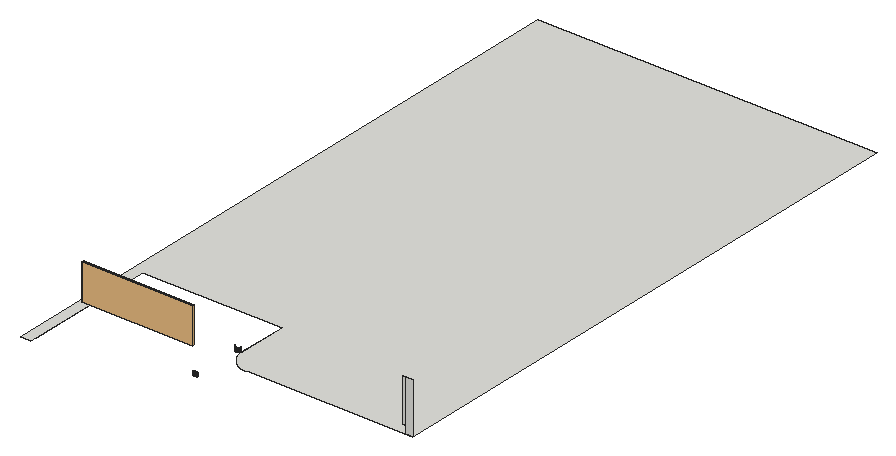
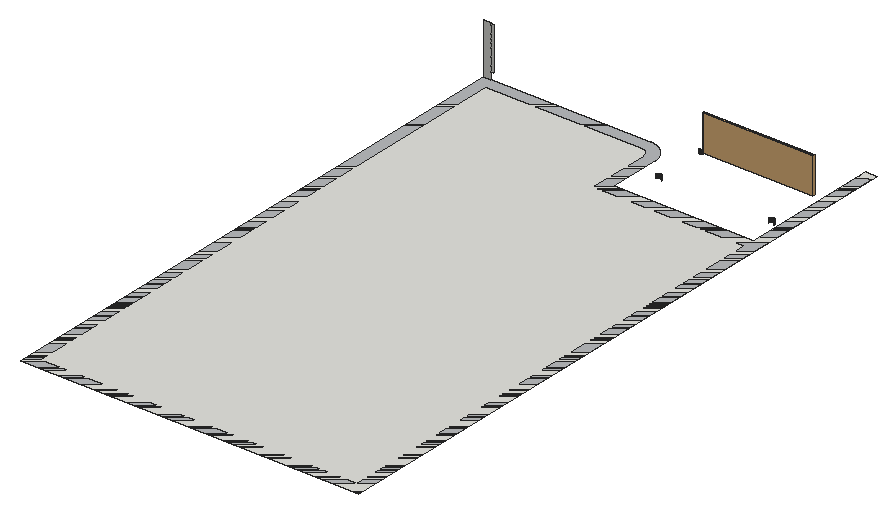
# SketchUp Ruby script. Lengths in inches.
U = 1.inch
M = Sketchup.active_model
def pt(a) = Geom::Point3d.new(a.map { |v| v * U })
def face(e, loops, mat)
  f = e.add_face(loops[0].map { |a| pt(a) })
  loops[1..].each { |l| e.add_face(l.map { |a| pt(a) }).erase! }
  f.material = f.back_material = mat if mat
  f
end
# faces: each face lists its corners as indices into pts; further lists are holes
def faces(e, pts, list, mat = nil) = list.each { |f| face(e, (f[0].is_a?(Array) ? f : [f]).map { |l| l.map { |i| pts[i] } }, mat) }
# xy, xz, yz: faces in a plane at the given z, y or x. An outline is a flat list of corners, or four numbers for a rectangle; further outlines are holes
def ring(l) = l.size == 4 ? [[l[0], l[1]], [l[2], l[1]], [l[2], l[3]], [l[0], l[3]]] : l.each_slice(2).to_a
def flat(e, list, mat, &to3) = list.each { |f| face(e, (f[0].is_a?(Array) ? f : [f]).map { |l| ring(l).map { |u, v| to3.(u, v) } }, mat) }
def xy(e, z, list, mat = nil) = flat(e, list, mat) { |x, y| [x, y, z] }
def xz(e, y, list, mat = nil) = flat(e, list, mat) { |x, z| [x, y, z] }
def yz(e, x, list, mat = nil) = flat(e, list, mat) { |y, z| [x, y, z] }
def lines(e, pts, list) = list.each { |a, b| e.add_line(pt(pts[a]), pt(pts[b])) }
# prism: a flat outline (further loops are holes) pulled along v
def prism(e, loops, v, mat = nil)
  f = face(e, loops, mat); d = Geom::Vector3d.new(v.map { |x| x * U })
  f.pushpull(f.normal.samedirection?(d) ? d.length : -d.length)
end
def box(e, o, s, mat = nil) = prism(e, [[o, [o[0] + s[0], o[1], o[2]], [o[0] + s[0], o[1] + s[1], o[2]], [o[0], o[1] + s[1], o[2]]]], [0, 0, s[2]], mat)
def at(x, y, z, deg = 0) = Geom::Transformation.translation(pt([x, y, z])) * Geom::Transformation.rotation(ORIGIN, Z_AXIS, deg.degrees)
def axes(o, x, y, z) = Geom::Transformation.new([*x, 0, *y, 0, *z, 0, *pt(o).to_a, 1])
def part(name) = M.definitions.add(name)
# library, detail: a bought-in or finely detailed component or shape, given as its bounding box
def library(name, o, s) = part(name).tap { |d| box(d.entities, o, s) }
def detail(e, o, s) = box(e.add_group.entities, o, s)
def put(e, d, t, mat = nil) = e.add_instance(d, t).tap { |i| i.material = mat if mat }
def group(e, t, mat = nil) = e.add_group.tap { |g| g.transformation = t; g.material = mat if mat }.entities
root = M.entities
M.materials.add("1427 AP 686 ARMOUR-N").color = [184, 186, 189]
M.materials.add("[Wood Veneer 01]").color = [99, 65, 43]
c1 = library("Group\#10",[-36,0,0],[116,2,29.75])
xy(root,372,[[9,135.92,9,672,290,672,290,192,151.76,192,151.53,192.01,151.29,192.01,151.06,192.02,150.82,192.04,150.59,192.06,150.35,192.08,150.12,192.1,149.88,192.125,149.65,192.15,149.42,192.1875,149.18,192.22,148.72,192.3,148.49,192.35,148.26,192.39,148.03,192.44,147.8,192.5,147.57,192.55,147.34,192.61,147.11,192.68,146.89,192.74,146.66,192.81,146.4375,192.88,146.21,192.96,145.99,193.03,145.77,193.11,145.55,193.2,145.33,193.28,144.89,193.46,144.68,193.56,144.46,193.65,144.25,193.75,144.04,193.86,143.83,193.96,143.41,194.18,143.2,194.3,143,194.41,142.6,194.65,142.39,194.78,142.2,194.9,142,195.03,141.8,195.17,141.61,195.3,141.42,195.4375,141.23,195.58,141.04,195.72,140.86,195.86,140.67,196.01,140.49,196.16,140.31,196.3125,140.13,196.47,139.96,196.625,139.78,196.78,139.61,196.94,139.44,197.11,139.27,197.27,139.11,197.44,138.94,197.61,138.78,197.78,138.625,197.96,138.47,198.13,138.3125,198.31,138.16,198.49,138.01,198.67,137.86,198.86,137.72,199.04,137.58,199.23,137.4375,199.42,137.3,199.61,137.17,199.8,137.03,200,136.9,200.2,136.78,200.39,136.65,200.6,136.41,201,136.3,201.2,136.18,201.41,135.96,201.83,135.86,202.04,135.75,202.25,135.65,202.46,135.56,202.68,135.46,202.89,135.28,203.33,135.2,203.55,135.11,203.77,135.03,203.99,134.96,204.21,134.88,204.4375,134.81,204.66,134.74,204.89,134.68,205.11,134.61,205.34,134.55,205.57,134.5,205.8,134.44,206.03,134.39,206.26,134.35,206.49,134.3,206.72,134.22,207.18,134.1875,207.42,134.15,207.65,134.125,207.88,134.1,208.12,134.08,208.35,134.06,208.59,134.04,208.82,134.02,209.06,134.01,209.29,134.01,209.53,134,209.76,134,252,18,252,18,135.92]])
xy(root,372,[[[9,141.92,18,141.92,18,252,134,252,134,209.78,134.01,209.57,134.01,209.35,134.03,208.91,134.05,208.7,134.0625,208.48,134.08,208.26,134.11,208.05,134.13,207.83,134.16,207.61,134.1875,207.4,134.22,207.18,134.26,206.97,134.29,206.76,134.34,206.54,134.42,206.12,134.47,205.9,134.52,205.69,134.58,205.48,134.63,205.27,134.69,205.0625,134.75,204.85,134.82,204.64,134.88,204.4375,134.95,204.23,135.02,204.03,135.09,203.82,135.17,203.62,135.25,203.41,135.41,203.01,135.5,202.8125,135.59,202.61,135.68,202.41,135.77,202.22,135.86,202.02,135.96,201.83,136.0625,201.63,136.16,201.44,136.27,201.25,136.48,200.875,136.6,200.6875,136.71,200.5,136.83,200.32,136.94,200.14,137.0625,199.95,137.1875,199.77,137.3125,199.6,137.4375,199.42,137.57,199.24,137.83,198.9,137.97,198.73,138.1,198.56,138.24,198.39,138.38,198.23,138.53,198.0625,138.67,197.9,138.97,197.58,139.12,197.43,139.27,197.27,139.43,197.12,139.58,196.97,139.9,196.67,140.0625,196.53,140.23,196.38,140.39,196.24,140.56,196.1,140.73,195.97,140.9,195.83,141.24,195.57,141.42,195.4375,141.6,195.3125,141.77,195.1875,141.95,195.0625,142.14,194.94,142.32,194.83,142.5,194.71,142.6875,194.6,142.875,194.48,143.25,194.27,143.44,194.16,143.63,194.0625,143.83,193.96,144.02,193.86,144.22,193.77,144.41,193.68,144.61,193.59,144.8125,193.5,145.01,193.41,145.41,193.25,145.62,193.17,145.82,193.09,146.03,193.02,146.23,192.95,146.4375,192.88,146.64,192.82,146.85,192.75,147.0625,192.69,147.27,192.63,147.48,192.58,147.69,192.52,147.9,192.47,148.12,192.42,148.54,192.34,148.76,192.29,148.97,192.26,149.18,192.22,149.4,192.1875,149.61,192.16,149.83,192.13,150.05,192.11,150.26,192.08,150.48,192.0625,150.7,192.05,150.91,192.03,151.35,192.01,151.57,192.01,151.78,192,290,192,290,672,9,672],[151.78,201,151.67,201.01,151.57,201.01,151.46,201.02,151.35,201.02,151.02,201.05,150.92,201.07,150.7,201.09,150.48,201.13,150.38,201.15,150.27,201.17,150.16,201.1875,150.06,201.21,149.95,201.24,149.85,201.26,149.74,201.29,149.64,201.32,149.53,201.35,149.43,201.375,149.32,201.41,149.12,201.47,149.01,201.51,148.91,201.55,148.81,201.58,148.71,201.625,148.61,201.66,148.51,201.71,148.31,201.79,148.21,201.84,148.11,201.88,147.91,201.98,147.82,202.03,147.72,202.08,147.625,202.13,147.53,202.1875,147.4375,202.24,147.34,202.3,147.25,202.35,146.89,202.59,146.8,202.66,146.62,202.78,146.54,202.85,146.45,202.92,146.36,202.98,146.2,203.12,146.11,203.19,146.03,203.26,145.95,203.34,145.79,203.48,145.71,203.56,145.64,203.64,145.56,203.71,145.48,203.79,145.34,203.95,145.26,204.03,145.19,204.11,145.12,204.2,144.98,204.36,144.92,204.45,144.85,204.54,144.78,204.62,144.66,204.8,144.59,204.89,144.35,205.25,144.3,205.34,144.24,205.4375,144.1875,205.53,144.13,205.625,144.08,205.72,144.03,205.82,143.98,205.91,143.88,206.11,143.84,206.21,143.79,206.31,143.71,206.51,143.66,206.61,143.625,206.71,143.58,206.81,143.55,206.91,143.51,207.01,143.47,207.12,143.41,207.32,143.375,207.43,143.35,207.53,143.32,207.64,143.29,207.74,143.26,207.85,143.24,207.95,143.21,208.06,143.1875,208.16,143.17,208.27,143.15,208.38,143.13,208.48,143.09,208.7,143.07,208.92,143.05,209.02,143.02,209.35,143.02,209.46,143.01,209.57,143.01,209.67,143,209.78,143,261,18,261,18,663,281,663,281,201]]],"1427 AP 686 ARMOUR-N")
xz(root,175.25,[[123.09,366,123.17,369],[123.17,366,123.25,369],[123.25,366,123.33,369],[123.33,366,123.41,369]])
xz(root,192,[[284,372,290,414],[281,378,284,414]])
xz(root,216.5,[[29.84,366,29.92,369],[29.92,366,30,369],[30,366,30.08,369],[30.08,366,30.16,369],[123.09,366,123.17,369],
  [123.17,366,123.25,369],[123.25,366,123.33,369],[123.33,366,123.41,369]])
p = [[121.48,174.52,366],[121.54,174.57,366],[121.54,174.57,369],[121.48,174.52,369],[124.96,174.57,366],[125.02,174.52,366],
  [125.02,174.52,369],[124.96,174.57,369],[121.6,174.625,366],[121.6,174.625,369],[121.66,174.68,366],[121.66,174.68,369],
  [124.84,174.68,366],[124.9,174.625,366],[124.9,174.625,369],[124.84,174.68,369],[121.72,174.73,366],[121.72,174.73,369],
  [121.78,174.77,366],[121.78,174.77,369],[124.72,174.77,366],[124.78,174.73,366],[124.78,174.73,369],[124.72,174.77,369],
  [121.84,174.82,366],[121.84,174.82,369],[121.91,174.86,366],[121.91,174.86,369],[124.59,174.86,366],[124.66,174.82,366],
  [124.66,174.82,369],[124.59,174.86,369],[121.98,174.9,366],[121.98,174.9,369],[122.05,174.94,366],[122.05,174.94,369],
  [122.12,174.98,366],[122.12,174.98,369],[124.38,174.98,366],[124.45,174.94,366],[124.45,174.94,369],[124.38,174.98,369],
  [124.52,174.9,366],[124.52,174.9,369],[122.1875,175.01,366],[122.1875,175.01,369],[122.26,175.04,366],[122.26,175.04,369],
  [122.33,175.07,366],[122.33,175.07,369],[124.24,175.04,366],[124.3125,175.01,366],[124.3125,175.01,369],[124.24,175.04,369],
  [124.17,175.07,366],[124.17,175.07,369],[122.4,175.1,366],[122.4,175.1,369],[122.48,175.13,366],[122.48,175.13,369],
  [122.55,175.15,366],[122.55,175.15,369],[123.95,175.15,366],[124.02,175.13,366],[124.02,175.13,369],[123.95,175.15,369],
  [124.1,175.1,366],[124.1,175.1,369],[122.63,175.17,366],[122.63,175.17,369],[122.7,175.19,366],[122.7,175.19,369],
  [122.78,175.21,366],[122.78,175.21,369],[122.86,175.22,366],[122.86,175.22,369],[122.9375,175.23,366],[122.9375,175.23,369],
  [123.01,175.24,366],[123.01,175.24,369],[123.09,175.25,366],[123.09,175.25,369],[123.41,175.25,366],[123.49,175.24,366],
  [123.49,175.24,369],[123.41,175.25,369],[123.5625,175.23,366],[123.5625,175.23,369],[123.64,175.22,366],[123.72,175.21,366],
  [123.72,175.21,369],[123.64,175.22,369],[123.8,175.19,366],[123.8,175.19,369],[123.87,175.17,366],[123.87,175.17,369],
  [29.61,216.53,366],[29.53,216.54,366],[29.53,216.54,369],[29.61,216.53,369],[29.45,216.56,366],[29.45,216.56,369],
  [29.6875,216.52,366],[29.6875,216.52,369],[29.76,216.51,366],[29.76,216.51,369],[29.84,216.5,366],[29.84,216.5,369],
  [30.24,216.51,366],[30.16,216.5,366],[30.16,216.5,369],[30.24,216.51,369],[30.3125,216.52,366],[30.3125,216.52,369],
  [30.39,216.53,366],[30.39,216.53,369],[30.47,216.54,366],[30.47,216.54,369],[30.55,216.56,366],[30.55,216.56,369],
  [122.78,216.54,366],[122.7,216.56,366],[122.7,216.56,369],[122.78,216.54,369],[122.86,216.53,366],[122.86,216.53,369],
  [123.01,216.51,366],[122.9375,216.52,366],[122.9375,216.52,369],[123.01,216.51,369],[123.09,216.5,366],[123.09,216.5,369],
  [123.49,216.51,366],[123.41,216.5,366],[123.41,216.5,369],[123.49,216.51,369],[123.5625,216.52,366],[123.5625,216.52,369],
  [123.64,216.53,366],[123.64,216.53,369],[123.72,216.54,366],[123.72,216.54,369],[123.8,216.56,366],[123.8,216.56,369],
  [29.15,216.65,366],[29.08,216.68,366],[29.08,216.68,369],[29.15,216.65,369],[29.3,216.6,366],[29.23,216.62,366],
  [29.23,216.62,369],[29.3,216.6,369],[29.38,216.58,366],[29.38,216.58,369],[30.62,216.58,366],[30.62,216.58,369],
  [30.7,216.6,366],[30.7,216.6,369],[30.77,216.62,366],[30.77,216.62,369],[30.85,216.65,366],[30.85,216.65,369],
  [30.92,216.68,366],[30.92,216.68,369],[122.4,216.65,366],[122.33,216.68,366],[122.33,216.68,369],[122.4,216.65,369],
  [122.48,216.62,366],[122.48,216.62,369],[122.55,216.6,366],[122.55,216.6,369],[122.63,216.58,366],[122.63,216.58,369],
  [123.87,216.58,366],[123.87,216.58,369],[123.95,216.6,366],[123.95,216.6,369],[124.02,216.62,366],[124.02,216.62,369],
  [124.1,216.65,366],[124.1,216.65,369],[124.17,216.68,366],[124.17,216.68,369],[29.01,216.71,366],[28.9375,216.74,366],
  [28.9375,216.74,369],[29.01,216.71,369],[28.87,216.77,366],[28.87,216.77,369],[30.99,216.71,366],[30.99,216.71,369],
  [31.0625,216.74,366],[31.0625,216.74,369],[31.13,216.77,366],[31.13,216.77,369],[122.1875,216.74,366],[122.12,216.77,366],
  [122.12,216.77,369],[122.1875,216.74,369],[122.26,216.71,366],[122.26,216.71,369],[124.24,216.71,366],[124.24,216.71,369],
  [124.3125,216.74,366],[124.3125,216.74,369],[124.38,216.77,366],[124.38,216.77,369],[28.8,216.81,366],[28.73,216.85,366],
  [28.73,216.85,369],[28.8,216.81,369],[28.66,216.89,366],[28.66,216.89,369],[31.2,216.81,366],[31.2,216.81,369],
  [31.27,216.85,366],[31.27,216.85,369],[31.34,216.89,366],[31.34,216.89,369],[121.98,216.85,366],[121.91,216.89,366],
  [121.91,216.89,369],[121.98,216.85,369],[122.05,216.81,366],[122.05,216.81,369],[124.45,216.81,366],[124.45,216.81,369],
  [124.52,216.85,366],[124.52,216.85,369],[124.59,216.89,366],[124.59,216.89,369],[28.59,216.93,366],[28.53,216.98,366],
  [28.53,216.98,369],[28.59,216.93,369],[31.41,216.93,366],[31.41,216.93,369],[31.47,216.98,366],[31.47,216.98,369],
  [121.84,216.93,366],[121.84,216.93,369],[121.78,216.98,366],[121.78,216.98,369],[124.66,216.93,366],[124.66,216.93,369],
  [124.72,216.98,366],[124.72,216.98,369],[28.47,217.02,366],[28.41,217.07,366],[28.41,217.07,369],[28.47,217.02,369],
  [31.53,217.02,366],[31.53,217.02,369],[31.59,217.07,366],[31.59,217.07,369],[121.72,217.02,366],[121.72,217.02,369],
  [121.66,217.07,366],[121.66,217.07,369],[124.78,217.02,366],[124.78,217.02,369],[124.84,217.07,366],[124.84,217.07,369],
  [28.35,217.125,366],[28.35,217.125,369],[28.29,217.18,366],[28.29,217.18,369],[31.65,217.125,366],[31.65,217.125,369],
  [31.71,217.18,366],[31.71,217.18,369],[121.6,217.125,366],[121.54,217.18,366],[121.54,217.18,369],[121.6,217.125,369],
  [124.9,217.125,366],[124.9,217.125,369],[124.96,217.18,366],[124.96,217.18,369],[28.23,217.23,366],[28.23,217.23,369],
  [28.18,217.29,366],[28.18,217.29,369],[31.77,217.23,366],[31.77,217.23,369],[31.82,217.29,366],[31.82,217.29,369],
  [121.48,217.23,366],[121.43,217.29,366],[121.43,217.29,369],[121.48,217.23,369],[125.02,217.23,366],[125.02,217.23,369],
  [125.07,217.29,366],[125.07,217.29,369],[28.125,217.35,366],[28.125,217.35,369],[28.07,217.41,366],[28.07,217.41,369],
  [31.875,217.35,366],[31.875,217.35,369],[31.93,217.41,366],[31.93,217.41,369],[121.375,217.35,366],[121.32,217.41,366],
  [121.32,217.41,369],[121.375,217.35,369],[125.125,217.35,366],[125.125,217.35,369],[125.18,217.41,366],[125.18,217.41,369],
  [28.02,217.47,366],[28.02,217.47,369],[31.98,217.47,366],[31.98,217.47,369],[121.27,217.47,366],[121.27,217.47,369],
  [125.23,217.47,366],[125.23,217.47,369],[27.98,217.53,366],[27.93,217.59,366],[27.93,217.59,369],[27.98,217.53,369],
  [32.02,217.53,366],[32.02,217.53,369],[32.07,217.59,366],[32.07,217.59,369],[121.23,217.53,366],[121.23,217.53,369],
  [121.18,217.59,366],[121.18,217.59,369],[125.27,217.53,366],[125.27,217.53,369],[125.32,217.59,366],[125.32,217.59,369],
  [27.89,217.66,366],[27.89,217.66,369],[32.11,217.66,366],[32.11,217.66,369],[121.14,217.66,366],[121.14,217.66,369],
  [125.36,217.66,366],[125.36,217.66,369],[27.85,217.73,366],[27.85,217.73,369],[27.81,217.8,366],[27.81,217.8,369],
  [32.15,217.73,366],[32.15,217.73,369],[32.19,217.8,366],[32.19,217.8,369],[121.1,217.73,366],[121.1,217.73,369],
  [121.06,217.8,366],[121.06,217.8,369],[125.4,217.73,366],[125.4,217.73,369],[125.44,217.8,366],[125.44,217.8,369],
  [27.77,217.87,366],[27.77,217.87,369],[32.23,217.87,366],[32.23,217.87,369],[121.02,217.87,366],[121.02,217.87,369],
  [125.48,217.87,366],[125.48,217.87,369],[27.74,217.9375,366],[27.74,217.9375,369],[27.71,218.01,366],[27.71,218.01,369],
  [32.26,217.9375,366],[32.26,217.9375,369],[32.29,218.01,366],[32.29,218.01,369],[120.99,217.9375,366],[120.99,217.9375,369],
  [120.96,218.01,366],[120.96,218.01,369],[125.51,217.9375,366],[125.51,217.9375,369],[125.54,218.01,366],[125.54,218.01,369],
  [27.68,218.08,366],[27.68,218.08,369],[32.32,218.08,366],[32.32,218.08,369],[120.93,218.08,366],[120.93,218.08,369],
  [125.57,218.08,366],[125.57,218.08,369],[27.65,218.15,366],[27.65,218.15,369],[32.35,218.15,366],[32.35,218.15,369],
  [120.9,218.15,366],[120.9,218.15,369],[125.6,218.15,366],[125.6,218.15,369],[27.62,218.23,366],[27.62,218.23,369],
  [27.6,218.3,366],[27.6,218.3,369],[32.38,218.23,366],[32.38,218.23,369],[32.4,218.3,366],[32.4,218.3,369],
  [120.87,218.23,366],[120.85,218.3,366],[120.85,218.3,369],[120.87,218.23,369],[125.63,218.23,366],[125.63,218.23,369],
  [125.65,218.3,366],[125.65,218.3,369],[27.58,218.38,366],[27.58,218.38,369],[32.42,218.38,366],[32.42,218.38,369],
  [120.83,218.38,366],[120.83,218.38,369],[125.67,218.38,366],[125.67,218.38,369],[27.56,218.45,366],[27.56,218.45,369],
  [32.44,218.45,366],[32.44,218.45,369],[120.81,218.45,366],[120.81,218.45,369],[125.69,218.45,366],[125.69,218.45,369],
  [27.54,218.53,366],[27.54,218.53,369],[32.46,218.53,366],[32.46,218.53,369],[120.79,218.53,366],[120.79,218.53,369],
  [125.71,218.53,366],[125.71,218.53,369],[125.72,218.61,366],[125.72,218.61,369]]
faces(root,p,[[0,1,2,3],[4,5,6,7],[1,8,9,2],[8,10,11,9],[12,13,14,15],[13,4,7,14],[10,16,17,11],[16,18,19,17],
  [20,21,22,23],[21,12,15,22],[18,24,25,19],[24,26,27,25],[28,29,30,31],[29,20,23,30],[26,32,33,27],[32,34,35,33],
  [34,36,37,35],[38,39,40,41],[42,28,31,43],[39,42,43,40],[36,44,45,37],[44,46,47,45],[46,48,49,47],[50,51,52,53],
  [54,50,53,55],[51,38,41,52],[48,56,57,49],[56,58,59,57],[58,60,61,59],[62,63,64,65],[63,66,67,64],[66,54,55,67],
  [60,68,69,61],[68,70,71,69],[70,72,73,71],[72,74,75,73],[74,76,77,75],[76,78,79,77],[78,80,81,79],[82,83,84,85],
  [83,86,87,84],[88,89,90,91],[86,88,91,87],[89,92,93,90],[92,94,95,93],[94,62,65,95],[96,97,98,99],[97,100,101,98],
  [102,96,99,103],[104,102,103,105],[106,104,105,107],[108,109,110,111],[112,108,111,113],[114,112,113,115],[116,114,115,117],[118,116,117,119],
  [120,121,122,123],[124,120,123,125],[126,127,128,129],[127,124,125,128],[130,126,129,131],[132,133,134,135],[136,132,135,137],[138,136,137,139],
  [140,138,139,141],[142,140,141,143],[144,145,146,147],[148,149,150,151],[149,144,147,150],[152,148,151,153],[100,152,153,101],[154,118,119,155],
  [156,154,155,157],[158,156,157,159],[160,158,159,161],[162,160,161,163],[164,165,166,167],[168,164,167,169],[170,168,169,171],[121,172,173,122],
  [172,170,171,173],[174,142,143,175],[176,174,175,177],[178,176,177,179],[180,178,179,181],[182,180,181,183],[184,185,186,187],[185,188,189,186],
  [145,184,187,146],[190,162,163,191],[192,190,191,193],[194,192,193,195],[196,197,198,199],[200,196,199,201],[165,200,201,166],[202,182,183,203],
  [204,202,203,205],[206,204,205,207],[208,209,210,211],[209,212,213,210],[188,208,211,189],[214,194,195,215],[216,214,215,217],[218,216,217,219],
  [220,221,222,223],[197,224,225,198],[224,220,223,225],[226,206,207,227],[228,226,227,229],[230,228,229,231],[232,233,234,235],[212,232,235,213],
  [236,218,219,237],[238,236,237,239],[221,240,241,222],[240,242,243,241],[244,230,231,245],[246,244,245,247],[248,249,250,251],[233,248,251,234],
  [252,238,239,253],[254,252,253,255],[242,256,257,243],[256,258,259,257],[260,246,247,261],[262,260,261,263],[249,264,265,250],[264,266,267,265],
  [268,254,255,269],[270,268,269,271],[272,273,274,275],[258,272,275,259],[276,262,263,277],[278,276,277,279],[266,280,281,267],[280,282,283,281],
  [284,270,271,285],[286,284,285,287],[288,289,290,291],[273,288,291,274],[292,278,279,293],[294,292,293,295],[282,296,297,283],[296,298,299,297],
  [300,286,287,301],[302,300,301,303],[304,305,306,307],[289,304,307,290],[308,294,295,309],[310,308,309,311],[298,312,313,299],[314,302,303,315],
  [305,316,317,306],[318,310,311,319],[320,321,322,323],[312,320,323,313],[324,314,315,325],[326,324,325,327],[316,328,329,317],[328,330,331,329],
  [332,318,319,333],[334,332,333,335],[321,336,337,322],[338,326,327,339],[330,340,341,331],[342,334,335,343],[336,344,345,337],[344,346,347,345],
  [348,338,339,349],[350,348,349,351],[340,352,353,341],[352,354,355,353],[356,342,343,357],[358,356,357,359],[346,360,361,347],[362,350,351,363],
  [354,364,365,355],[366,358,359,367],[360,368,369,361],[368,370,371,369],[372,362,363,373],[374,372,373,375],[364,376,377,365],[376,378,379,377],
  [380,366,367,381],[382,380,381,383],[370,384,385,371],[386,374,375,387],[378,388,389,379],[390,382,383,391],[384,392,393,385],[394,386,387,395],
  [388,396,397,389],[398,390,391,399],[392,400,401,393],[400,402,403,401],[404,394,395,405],[406,404,405,407],[408,409,410,411],[396,408,411,397],
  [412,398,399,413],[414,412,413,415],[402,416,417,403],[418,406,407,419],[409,420,421,410],[422,414,415,423],[416,424,425,417],[426,418,419,427],
  [420,428,429,421],[430,422,423,431],[424,432,433,425],[434,426,427,435],[428,436,437,429],[438,430,431,439],[440,438,439,441]])
put(root,c1,axes([46.55,188,378],[0.7931,0,0],[0,1,0],[0,0,1]),"[Wood Veneer 01]")
